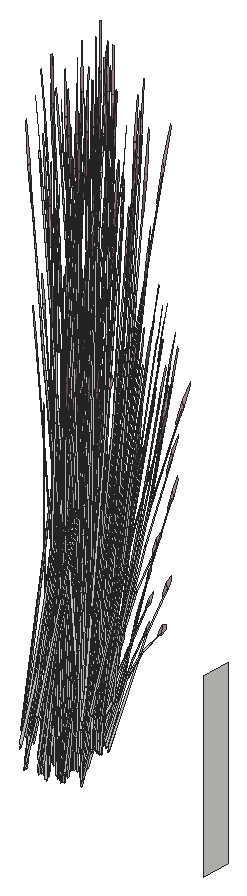
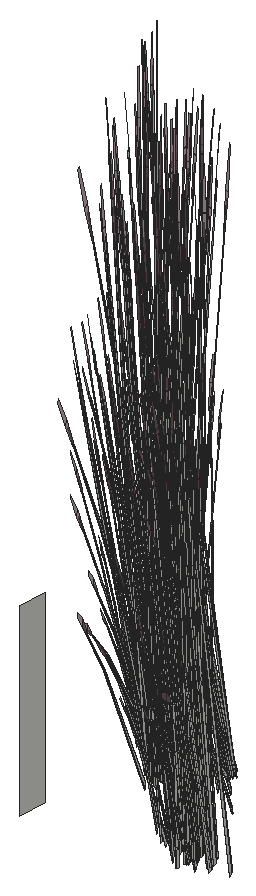
# SketchUp Ruby script. Lengths in inches.
U = 1.inch
M = Sketchup.active_model
def pt(a) = Geom::Point3d.new(a.map { |v| v * U })
def face(e, loops, mat)
  f = e.add_face(loops[0].map { |a| pt(a) })
  loops[1..].each { |l| e.add_face(l.map { |a| pt(a) }).erase! }
  f.material = f.back_material = mat if mat
  f
end
# faces: each face lists its corners as indices into pts; further lists are holes
def faces(e, pts, list, mat = nil) = list.each { |f| face(e, (f[0].is_a?(Array) ? f : [f]).map { |l| l.map { |i| pts[i] } }, mat) }
# xy, xz, yz: faces in a plane at the given z, y or x. An outline is a flat list of corners, or four numbers for a rectangle; further outlines are holes
def ring(l) = l.size == 4 ? [[l[0], l[1]], [l[2], l[1]], [l[2], l[3]], [l[0], l[3]]] : l.each_slice(2).to_a
def flat(e, list, mat, &to3) = list.each { |f| face(e, (f[0].is_a?(Array) ? f : [f]).map { |l| ring(l).map { |u, v| to3.(u, v) } }, mat) }
def xy(e, z, list, mat = nil) = flat(e, list, mat) { |x, y| [x, y, z] }
def xz(e, y, list, mat = nil) = flat(e, list, mat) { |x, z| [x, y, z] }
def yz(e, x, list, mat = nil) = flat(e, list, mat) { |y, z| [x, y, z] }
def lines(e, pts, list) = list.each { |a, b| e.add_line(pt(pts[a]), pt(pts[b])) }
# prism: a flat outline (further loops are holes) pulled along v
def prism(e, loops, v, mat = nil)
  f = face(e, loops, mat); d = Geom::Vector3d.new(v.map { |x| x * U })
  f.pushpull(f.normal.samedirection?(d) ? d.length : -d.length)
end
def box(e, o, s, mat = nil) = prism(e, [[o, [o[0] + s[0], o[1], o[2]], [o[0] + s[0], o[1] + s[1], o[2]], [o[0], o[1] + s[1], o[2]]]], [0, 0, s[2]], mat)
def at(x, y, z, deg = 0) = Geom::Transformation.translation(pt([x, y, z])) * Geom::Transformation.rotation(ORIGIN, Z_AXIS, deg.degrees)
def axes(o, x, y, z) = Geom::Transformation.new([*x, 0, *y, 0, *z, 0, *pt(o).to_a, 1])
def part(name) = M.definitions.add(name)
# library, detail: a bought-in or finely detailed component or shape, given as its bounding box
def library(name, o, s) = part(name).tap { |d| box(d.entities, o, s) }
def detail(e, o, s) = box(e.add_group.entities, o, s)
def put(e, d, t, mat = nil) = e.add_instance(d, t).tap { |i| i.material = mat if mat }
def group(e, t, mat = nil) = e.add_group.tap { |g| g.transformation = t; g.material = mat if mat }.entities
root = M.entities
M.materials.add("LightPink_Translucent").color = [144, 107, 117]
M.materials["LightPink_Translucent"].alpha = 0.75
c1 = part("blade")
p = [[2.15,0.21,22],[0,0.17,0],[0.09,0.45,0],[2.18,0.31,22],[2.29,0.31,22],[0.38,0.45,0],
  [2.48,0.24,33],[2.49,0.24,33],[2.48,0.22,33]]
faces(c1.entities,p,[[0,1,2,3],[4,5,2,3],[6,3,4,7],[8,0,3,6]])
c2 = part("seeds")
p = [[0.3,-0.1,1.38],[-0.01,-0.03,1.59],[-0.01,-0.03,0.03],[0.14,-0.07,-0.07],[0.29,-0.03,3],[0.15,0.01,3.11]]
faces(c2.entities,p,[[0,1,2,3],[1,0,4,5]],"LightPink_Translucent")
c3 = part("blade with seeds")
put(c3.entities,c1,at(0,0,0))
put(c3.entities,c2,axes([2.4,0.25,30.99],[1.5799,-0.05474,1.17369],[-0.12525,1.92788,0.29478],[-0.07173,-0.02425,1.56792]))
p = [[375.57,661.9,618],[375.4,659.16,618],[375.4,659.16,636],[375.57,661.9,636]]
faces(root,p,[[0,1,2,3]])
put(root,c3,axes([358.46,657.71,625.58],[-0.26007,0.1585,0.0643],[-0.12729,-0.28902,0.50621],[0.02512,0.1274,0.77189]))
put(root,c3,axes([360.16,659.93,627.39],[0.04504,0.01251,1.77383],[0.13934,0.41205,-0.16761],[-0.0922,0.10815,0.31391]))
put(root,c3,axes([361.1875,659.42,627.36],[-0.09562,0.42421,-0.51099],[-0.32782,-0.1454,-0.3958],[-0.13199,0.0389,0.97773]))
put(root,c3,axes([357.42,661.35,620.03],[0.08291,0.40636,-0.30978],[-0.32928,0.11539,0.30978],[0.06638,0.04686,1.38974]))
put(root,c3,axes([356.62,662,620.67],[0.35635,-0.30962,-0.29095],[0.23697,0.43749,-0.50002],[0.08792,0.04443,1.59708]))
put(root,c3,axes([359.68,662.6,620.47],[-0.2773,-0.3397,0.17642],[0.27945,-0.32949,0.35086],[-0.03063,0.06937,1.60407]))
put(root,c3,axes([358.72,662.4,620.21],[0,-0.53961,0],[0.44133,0,0],[0,0,1.79456]))
put(root,c3,axes([357.68,661.94,623.05],[-0.30722,0.06665,0.35414],[-0.08112,-0.381,-0.4572],[0.08804,-0.10234,0.87481]))
put(root,c3,axes([360.54,661.24,625.45],[0.14709,-0.21136,1.1486],[0.05804,0.3346,0.84392],[-0.1063,0.05991,0.25299]))
put(root,c3,axes([358.31,662.5,620.43],[0.39767,0.22603,0.24065],[-0.19139,0.46966,0.50002],[0,-0.10827,1.60543]))
put(root,c3,axes([358.51,657.62,622.34],[0.05712,-0.02538,1.76342],[0.34359,0.13968,-0.26939],[0.01005,0.15742,0.30037]))
put(root,c3,axes([358.9375,662.61,620.29],[0,0.53934,-0.05637],[-0.44133,0,0],[0,0.01695,1.79368]))
put(root,c3,axes([358.18,662.18,620.72],[-0.38326,0.02879,0.44739],[-0.03466,-0.47788,-0.21531],[0.06861,-0.04843,1.43643]))
put(root,c3,axes([358.59,657.76,625.37],[-0.1064,0.35863,-0.35414],[-0.31043,-0.1046,0.4572],[0.02846,0.14439,0.87481]))
put(root,c3,axes([358,661.36,620.47],[-0.10196,0.46348,0.17642],[-0.3731,-0.13116,0.35086],[0.06445,-0.00226,1.60407]))
put(root,c3,axes([361.17,659.06,627.71],[0.17758,0.42229,-0.1216],[-0.31518,0.20752,-0.67495],[-0.13282,0.05572,1.02557]))
put(root,c3,axes([361.625,659.95,626.56],[0.08815,-0.14329,1.71376],[0.22258,0.38678,0.13857],[-0.15267,0.17614,0.73262]))
put(root,c3,axes([361.1,660.32,627.21],[-0.30722,0.06665,-0.35414],[-0.08112,-0.381,0.4572],[-0.08804,0.10234,0.87481]))
put(root,c3,axes([355.72,661.72,619.59],[-0.3474,0.18671,1.28929],[-0.11057,-0.53572,0.50096],[0.21332,0.00891,1.46642]))
put(root,c3,axes([360.93,661.45,624.17],[0.04734,0.04659,1.76342],[0.08027,0.4317,-0.26939],[-0.10492,0.09206,0.30037]))
put(root,c3,axes([358.37,658.4,625.56],[0.04474,0.0751,1.74944],[0.36104,0.0295,-0.27667],[0.03631,0.16562,0.14031]))
put(root,c3,axes([359.13,661.39,620.47],[-0.37926,0.12378,0.17642],[-0.09365,-0.46065,0.35086],[0.03382,0.06712,1.60407]))
put(root,c3,axes([357.31,660.89,620.375],[0.22066,-0.46731,0],[0.36918,0.26061,-0.51607],[0.08408,0.05936,1.63711]))
put(root,c3,axes([361.14,660.24,627.41],[-0.08753,-0.42921,0.48003],[0.34336,-0.07449,0.3958],[-0.1012,0.10094,0.9933]))
put(root,c3,axes([357.39,663.67,623.05],[-0.20082,-0.29199,0.35414],[0.2293,-0.2764,-0.4572],[0.1165,0.04206,0.87481]))
put(root,c3,axes([358.55,657.38,625.9],[0.1064,-0.35863,0.35414],[0.31043,0.1046,-0.4572],[0.02846,0.14439,0.87481]))
put(root,c3,axes([358.51,662.06,620.36],[-0.29264,0.42323,0.45755],[-0.34767,-0.3736,0.17955],[0.07055,-0.04224,1.58856]))
put(root,c3,axes([359.01,662.73,620.21],[0.24637,0.30123,0],[-0.24637,0.30123,0],[0,0,1.69266]))
put(root,c3,axes([357.52,661.17,620.02],[0.33032,0.23318,-0.49651],[-0.19744,0.41812,0],[0.07523,0.05311,1.57504]))
put(root,c3,axes([359,662.375,620.72],[0.17124,-0.42022,0.44739],[0.35581,0.20224,-0.21531],[0,0.09687,1.43643]))
put(root,c3,axes([361.07,660.16,627.41],[-0.2423,-0.19613,0.0643],[0.14107,-0.2793,0.50621],[-0.07768,0.0903,0.77189]))
put(root,c3,axes([358.89,662.27,620.38],[-0.44609,-0.09826,0.49198],[0.09078,-0.55493,0.19306],[0.06519,0.05359,1.70813]))
put(root,c3,axes([358.28,663.87,621.93],[-0.06755,-0.39203,-0.03492],[0.31928,-0.09013,-0.15832],[0.06667,0.02485,0.52218]))
put(root,c3,axes([357.72,662.86,623.05],[-0.29332,-0.1301,0.35414],[0.08555,-0.37955,-0.4572],[0.11809,-0.0348,0.87481]))
put(root,c3,axes([361.56,660.3,626.56],[0.06572,-0.16029,1.71376],[0.27569,0.33172,0.13857],[-0.12437,0.20675,0.73262]))
put(root,c3,axes([358.62,657.44,625.83],[0.16845,0.3792,-0.71045],[-0.34676,0.21133,0.08574],[0.03939,0.18322,1.00501]))
put(root,c3,axes([357.03,662.07,620.06],[0.36714,0.07646,-0.62353],[-0.07747,0.47163,-0.16365],[0.10956,0.05715,1.37633]))
put(root,c3,axes([358.6,662.35,620.26],[-0.21881,-0.29821,-0.06488],[0.23965,-0.27324,-0.29416],[0.0679,-0.01924,0.97024]))
put(root,c3,axes([361.3,659.1875,627.73],[0.29332,0.1301,0.35414],[-0.08555,0.37955,-0.4572],[-0.11809,0.0348,0.87481]))
put(root,c3,axes([359.02,662.52,620.21],[0.39487,0,0],[0,0.48281,0],[0,0,1.78407]))
put(root,c3,axes([361.35,660.37,627.36],[0.09067,0.42583,-0.51099],[-0.34336,0.07449,-0.3958],[-0.0984,0.11438,0.97773]))
put(root,c3,axes([358.64,661.99,620.72],[-0.21202,-0.39143,0.44739],[0.32115,-0.27564,-0.21531],[0.06861,0.04843,1.43643]))
put(root,c3,axes([358.25,662.08,620.67],[-0.04113,-0.53214,-0.29095],[0.42835,-0.03218,-0.50002],[0.07543,-0.07088,1.59708]))
put(root,c3,axes([359.15,662.47,620.62],[0.32884,-0.136,0.1448],[0.11516,0.38837,-0.41347],[0,0.08547,1.26744]))
put(root,c3,axes([358.97,658.66,626.49],[0.2439,-0.26754,-0.06488],[0.22348,0.29302,-0.29416],[0.01573,0.08303,0.97024]))
put(root,c3,axes([358.09,660.83,620.77],[-0.11756,0.2374,1.1486],[-0.10105,-0.31895,0.84392],[0.09709,-0.07992,0.25299]))
put(root,c3,axes([360.8125,661.13,627.4],[-0.00877,0.09229,1.74944],[0.24897,0.32105,-0.27667],[-0.06518,0.15182,0.14031]))
put(root,c3,axes([357.95,661.88,622.73],[0.2423,0.19613,0.0643],[-0.14107,0.2793,0.50621],[0.07768,-0.0903,0.77189]))
put(root,c3,axes([357.89,661.8,622.73],[0.08753,0.42921,0.48003],[-0.34336,0.07449,0.3958],[0.1012,-0.10094,0.9933]))
put(root,c3,axes([358.75,657.52,625.53],[0.34695,0.11691,-0.51099],[-0.11892,0.40083,-0.3958],[0.03181,0.16138,0.97773]))
put(root,c3,axes([358.45,657.54,625.88],[0.34538,-0.21713,-0.1216],[0.16972,0.38536,-0.67495],[0.04557,0.16239,1.02557]))
put(root,c3,axes([358.19,660.9,620.03],[0.32928,0.11539,-0.30978],[-0.08291,0.40636,0.30978],[0.06638,-0.04686,1.38974]))
put(root,c3,axes([358.64,661.87,622.71],[-0.0461,-0.00354,1.77383],[-0.19143,-0.37951,-0.16761],[0.07688,-0.12478,0.31391]))
put(root,c3,axes([361.72,660.96,624.7],[-0.33032,-0.23318,-0.49651],[0.19744,-0.41812,0],[-0.07523,-0.05311,1.57504]))
put(root,c3,axes([361.1875,660.0625,627.71],[0.32648,0.25715,-0.1216],[-0.18809,0.3724,-0.67495],[-0.09224,0.12945,1.02557]))
put(root,c3,axes([357.93,661.72,622.53],[0.30722,-0.06665,-0.35414],[0.08112,0.381,0.4572],[0.08804,-0.10234,0.87481]))
put(root,c3,axes([359.9,662.61,620.48],[0,-0.46636,0.49651],[0.39487,0,0],[0,0.10622,1.57504]))
put(root,c3,axes([358.12,660.72,620.02],[0.33032,-0.23318,-0.49651],[0.19744,0.41812,0],[0.07523,-0.05311,1.57504]))
put(root,c3,axes([361.92,661.24,625.05],[-0.22066,0.46731,0],[-0.36918,-0.26061,-0.51607],[-0.08408,-0.05936,1.63711]))
put(root,c3,axes([357.99,662.97,622.73],[0.12963,0.31798,0.0643],[-0.23638,0.15564,0.50621],[0.1042,-0.03071,0.77189]))
put(root,c3,axes([358.78,661.88,620.62],[0.06809,-0.4162,0.1448],[0.33266,0.07225,-0.41347],[0.06054,0.04274,1.26744]))
put(root,c3,axes([357.45,663.86,623.03],[0.0189,-0.47427,-0.1216],[0.35781,0.01296,-0.67495],[0.13781,0.03295,1.02557]))
put(root,c3,axes([357.85,662.98,623.03],[-0.17758,-0.42229,-0.1216],[0.31518,-0.20752,-0.67495],[0.13282,-0.05572,1.02557]))
put(root,c3,axes([357.97,662.86,622.73],[-0.09971,0.42522,0.48003],[-0.32782,-0.1454,0.3958],[0.12892,-0.02555,0.9933]))
put(root,c3,axes([360.65,661.18,628.33],[0.31145,0.12449,-0.06488],[-0.0958,0.38314,-0.29416],[-0.05094,0.05817,0.97024]))
put(root,c3,axes([359.25,661.15,620.48],[-0.33032,-0.23318,0.49651],[0.19744,-0.41812,0],[0.07523,0.05311,1.57504]))
put(root,c3,axes([361.35,660.1,627.73],[0.30722,-0.06665,0.35414],[0.08112,0.381,-0.4572],[-0.08804,0.10234,0.87481]))
put(root,c3,axes([358.96,663.59,620.18],[0.37054,-0.15823,-0.19198],[0.1302,0.45581,0.00008],[0.0409,-0.01749,1.73897]))
put(root,c3,axes([359.42,657.58,625.58],[-0.35104,0.10702,0.48003],[-0.06092,-0.41983,0.3958],[0.08256,0.12373,0.9933]))
put(root,c3,axes([359.35,657.67,625.58],[-0.16041,0.29625,0.0643],[-0.22843,-0.17248,0.50621],[0.07385,0.09498,0.77189]))
put(root,c3,axes([357.83,662.62,622.68],[0.09562,-0.42421,-0.51099],[0.32782,0.1454,-0.3958],[0.13199,-0.0389,0.97773]))
put(root,c3,axes([358.94,656.69,624.72],[-0.08068,-0.14973,1.71376],[0.3728,-0.12606,0.13857],[0.08426,0.23506,0.73262]))
put(root,c3,axes([358.97,662.23,620.21],[0.21202,0.39143,-0.44739],[-0.32115,0.27564,0.21531],[0.06861,0.04843,1.43643]))
put(root,c3,axes([358.66,662.89,620.77],[-0.21807,0.07699,1.1486],[0.10265,-0.31819,0.84392],[0.11568,0.02177,0.25299]))
put(root,c3,axes([362.62,660.13,625.35],[-0.35635,0.30962,-0.29095],[-0.23697,-0.43749,-0.50002],[-0.08792,-0.04443,1.59708]))
put(root,c3,axes([361.64,661.11,627.41],[-0.25132,-0.3182,0.48003],[0.2669,-0.27442,0.3958],[-0.04636,0.14929,0.9933]))
put(root,c3,axes([357.95,661.51,620.59],[-0.12609,-0.01381,1.43002],[-0.12917,-0.37055,-0.30754],[0.1549,-0.10482,0.61141]))
put(root,c3,axes([358.03,662.8125,622.53],[0.29332,0.1301,-0.35414],[-0.08555,0.37955,0.4572],[0.11809,-0.0348,0.87481]))
put(root,c3,axes([361.54,661.08,627.41],[-0.29004,-0.02173,0.0643],[0.00795,-0.32812,0.50621],[-0.03035,0.12569,0.77189]))
put(root,c3,axes([361.64,661.21,627.21],[-0.23881,0.24554,-0.35414],[-0.22606,-0.28036,0.4572],[-0.0344,0.14245,0.87481]))
put(root,c3,axes([358.51,661.67,620.06],[0.23773,-0.35053,-0.62353],[0.29532,0.31785,-0.16365],[0.09526,-0.08744,1.37633]))
put(root,c3,axes([362.86,660.47,624.74],[-0.23773,0.35053,-0.62353],[-0.29532,-0.31785,-0.16365],[-0.09526,0.08744,1.37633]))
put(root,c3,axes([358.18,662.74,619.98],[-0.22732,0.05597,1.41583],[-0.03618,-0.44548,0.08104],[0.15921,-0.06743,0.80566]))
put(root,c3,axes([358.43,662.45,619.49],[-0.01845,-0.0708,1.76342],[0.12793,-0.41416,-0.26939],[0.12905,-0.00596,0.30037]))
put(root,c3,axes([358.55,664.24,622.71],[-0.03191,-0.04083,1.77383],[0.06981,-0.43764,-0.16761],[0.12571,-0.02796,0.31391]))
put(root,c3,axes([359.55,661.36,620.03],[0.08291,0.40636,-0.30978],[-0.32928,0.11539,0.30978],[0.06638,0.04686,1.38974]))
put(root,c3,axes([357.23,662.34,621.875],[-0.14639,0.01056,1.71376],[0.09712,-0.45778,0.13857],[0.20862,0.02831,0.73262]))
put(root,c3,axes([358.75,662.01,620.67],[0.35635,-0.30962,-0.29095],[0.23697,0.43749,-0.50002],[0.08792,0.04443,1.59708]))
put(root,c3,axes([363.02,660.27,625.15],[-0.34464,-0.37536,-0.25192],[0.29,-0.42149,0.5513],[-0.0928,0.04391,1.68216]))
put(root,c3,axes([359.8,661.96,623.05],[-0.30722,0.06665,0.35414],[-0.08112,-0.381,-0.4572],[0.08804,-0.10234,0.87481]))
put(root,c3,axes([357.77,662.77,622.98],[0.31014,-0.20596,-0.71045],[0.17284,0.42397,0.08574],[0.14985,-0.04816,1.00501]))
put(root,c3,axes([359.26,656.99,623.4375],[0.00623,-0.15459,1.43002],[0.29764,-0.17268,-0.30754],[0.09188,0.18503,0.61141]))
put(root,c3,axes([362.85,660.19,624.89],[-0.38326,0.02879,-0.44739],[-0.03466,-0.47788,0.21531],[-0.06861,0.04843,1.43643]))
put(root,c3,axes([358.8125,662.32,622.72],[0.04898,-0.07104,1.74944],[-0.06269,-0.43574,-0.27667],[0.12289,-0.08262,0.14031]))
put(root,c3,axes([357.85,661.74,619.59],[-0.3474,0.18671,1.28929],[-0.11057,-0.53572,0.50096],[0.21332,0.00891,1.46642]))
put(root,c3,axes([362.11,660.99,625.16],[0.33032,0.23318,0.49651],[-0.19744,0.41812,0],[-0.07523,-0.05311,1.57504]))
put(root,c3,axes([358.25,663.4,620.59],[-0.085,-0.1147,1.43002],[0.1106,-0.37943,-0.30754],[0.17198,0.0514,0.61141]))
put(root,c3,axes([360,657.75,623.51],[-0.22633,-0.01463,1.0506],[0.14947,-0.31064,0.58006],[0.08941,0.11036,0.8241]))
put(root,c3,axes([362.59,660.27,625.3],[-0.06809,0.4162,0.1448],[-0.33266,-0.07225,-0.41347],[-0.06054,-0.04274,1.26744]))
put(root,c3,axes([359.44,660.91,620.375],[0.22066,-0.46731,0],[0.36918,0.26061,-0.51607],[0.08408,0.05936,1.63711]))
put(root,c3,axes([363.25,661.43,624.7],[-0.33032,0.23318,-0.49651],[-0.19744,-0.41812,0],[-0.07523,0.05311,1.57504]))
put(root,c3,axes([363.27,661.3,624.875],[-0.21791,-0.46895,-0.05142],[0.36918,-0.26061,0.51607],[-0.09097,0.04465,1.6363]))
put(root,c3,axes([359.52,663.69,623.05],[-0.20082,-0.29199,0.35414],[0.2293,-0.2764,-0.4572],[0.1165,0.04206,0.87481]))
put(root,c3,axes([359.64,661.19,620.02],[0.33032,0.23318,-0.49651],[-0.19744,0.41812,0],[0.07523,0.05311,1.57504]))
put(root,c3,axes([363.17,661.24,624.71],[-0.32928,-0.11539,-0.30978],[0.08291,-0.40636,0.30978],[-0.06638,0.04686,1.38974]))
put(root,c3,axes([361.76,660.86,627.73],[0.23881,-0.24554,0.35414],[0.22606,0.28036,-0.4572],[-0.0344,0.14245,0.87481]))
put(root,c3,axes([363.36,659.5,625.52],[-0.00964,-0.43909,1.41272],[0.43635,0.11382,0.59816],[-0.1032,0.24027,1.3335]))
put(root,c3,axes([360.41,663.89,621.93],[-0.06755,-0.39203,-0.03492],[0.31928,-0.09013,-0.15832],[0.06667,0.02485,0.52218]))
put(root,c3,axes([359.85,662.87,623.05],[-0.29332,-0.1301,0.35414],[0.08555,-0.37955,-0.4572],[0.11809,-0.0348,0.87481]))
put(root,c3,axes([359.16,662.08,620.06],[0.36714,0.07646,-0.62353],[-0.07747,0.47163,-0.16365],[0.10956,0.05715,1.37633]))
put(root,c3,axes([360.73,662.36,620.26],[-0.21881,-0.29821,-0.06488],[0.23965,-0.27324,-0.29416],[0.0679,-0.01924,0.97024]))
put(root,c3,axes([363.12,660.0625,625.35],[0.04113,0.53214,-0.29095],[-0.42835,0.03218,-0.50002],[-0.07543,0.07088,1.59708]))
put(root,c3,axes([359.52,657.32,625.53],[0.34827,-0.11086,-0.51099],[0.06092,0.41983,-0.3958],[0.09354,0.12031,0.97773]))
put(root,c3,axes([360.22,660.84,620.77],[-0.11756,0.2374,1.1486],[-0.10105,-0.31895,0.84392],[0.09709,-0.07992,0.25299]))
put(root,c3,axes([360.08,661.9,622.73],[0.2423,0.19613,0.0643],[-0.14107,0.2793,0.50621],[0.07768,-0.0903,0.77189]))
put(root,c3,axes([360.02,661.82,622.73],[0.08753,0.42921,0.48003],[-0.34336,0.07449,0.3958],[0.1012,-0.10094,0.9933]))
put(root,c3,axes([360.77,661.88,622.71],[-0.0461,-0.00354,1.77383],[-0.19143,-0.37951,-0.16761],[0.07688,-0.12478,0.31391]))
put(root,c3,axes([360.05,661.73,622.53],[0.30722,-0.06665,-0.35414],[0.08112,0.381,0.4572],[0.08804,-0.10234,0.87481]))
put(root,c3,axes([360.12,662.99,622.73],[0.12963,0.31798,0.0643],[-0.23638,0.15564,0.50621],[0.1042,-0.03071,0.77189]))
put(root,c3,axes([359.58,663.875,623.03],[0.0189,-0.47427,-0.1216],[0.35781,0.01296,-0.67495],[0.13781,0.03295,1.02557]))
put(root,c3,axes([359.98,663,623.03],[-0.17758,-0.42229,-0.1216],[0.31518,-0.20752,-0.67495],[0.13282,-0.05572,1.02557]))
put(root,c3,axes([362.24,660.76,625.15],[0.37926,-0.12378,0.17642],[0.09365,0.46065,0.35086],[-0.03382,-0.06712,1.60407]))
put(root,c3,axes([360.09,662.875,622.73],[-0.09971,0.42522,0.48003],[-0.32782,-0.1454,0.3958],[0.12892,-0.02555,0.9933]))
put(root,c3,axes([362.73,660.83,624.875],[-0.35581,-0.20937,0],[0.17124,-0.43505,0],[0,0,1.62707]))
put(root,c3,axes([363.55,661.35,625.05],[0.22066,0.46731,0],[-0.36918,0.26061,-0.51607],[-0.08408,0.05936,1.63711]))
put(root,c3,axes([362.33,661.59,627.41],[-0.26007,0.1585,0.0643],[-0.12729,-0.28902,0.50621],[0.02512,0.1274,0.77189]))
put(root,c3,axes([363.37,660.78,625.15],[0.10196,-0.46348,0.17642],[0.3731,0.13116,0.35086],[-0.06445,0.00226,1.60407]))
put(root,c3,axes([363.19,660.17,625.3],[0.26075,0.2802,0.1448],[-0.2175,0.31612,-0.41347],[-0.06054,0.04274,1.26744]))
put(root,c3,axes([363.1875,659.96,625.4],[0.38326,-0.02879,0.44739],[0.03466,0.47788,-0.21531],[-0.06861,0.04843,1.43643]))
put(root,c3,axes([359.96,662.64,622.68],[0.09562,-0.42421,-0.51099],[0.32782,0.1454,-0.3958],[0.13199,-0.0389,0.97773]))
put(root,c3,axes([363.28,661.0625,625.01],[0.44186,0.15158,0.30756],[-0.11054,0.54181,-0.36492],[-0.07313,0.06781,1.64885]))
put(root,c3,axes([360.78,662.91,620.77],[-0.21807,0.07699,1.1486],[0.10265,-0.31819,0.84392],[0.11568,0.02177,0.25299]))
put(root,c3,axes([363.47,661.03,625.16],[0.33032,-0.23318,0.49651],[0.19744,0.41812,0],[-0.07523,0.05311,1.57504]))
put(root,c3,axes([360.08,661.52,620.59],[-0.12609,-0.01381,1.43002],[-0.12917,-0.37055,-0.30754],[0.1549,-0.10482,0.61141]))
put(root,c3,axes([360.16,662.83,622.53],[0.29332,0.1301,-0.35414],[-0.08555,0.37955,0.4572],[0.11809,-0.0348,0.87481]))
put(root,c3,axes([362.81,660.65,624.88],[-0.11516,-0.40207,0],[0.32884,-0.1408,0],[0,0,1.54371]))
put(root,c3,axes([360.3125,662.76,619.98],[-0.22732,0.05597,1.41583],[-0.03618,-0.44548,0.08104],[0.15921,-0.06743,0.80566]))
put(root,c3,axes([360.56,662.46,619.49],[-0.01845,-0.0708,1.76342],[0.12793,-0.41416,-0.26939],[0.12905,-0.00596,0.30037]))
put(root,c3,axes([360.68,664.25,622.71],[-0.03191,-0.04083,1.77383],[0.06981,-0.43764,-0.16761],[0.12571,-0.02796,0.31391]))
put(root,c3,axes([359.36,662.36,621.875],[-0.14639,0.01056,1.71376],[0.09712,-0.45778,0.13857],[0.20862,0.02831,0.73262]))
put(root,c3,axes([363.27,659.86,624.89],[-0.17124,0.42022,-0.44739],[-0.35581,-0.20224,0.21531],[0,0.09687,1.43643]))
put(root,c3,axes([363.95,659.6,625.15],[-0.2773,-0.3397,0.17642],[0.27945,-0.32949,0.35086],[-0.03063,0.06937,1.60407]))
put(root,c3,axes([359.9,662.79,622.98],[0.31014,-0.20596,-0.71045],[0.17284,0.42397,0.08574],[0.14985,-0.04816,1.00501]))
put(root,c3,axes([363.21,659.62,624.97],[0,0.53934,-0.05637],[-0.44133,0,0],[0,0.01695,1.79368]))
put(root,c3,axes([362.43,661.26,627.73],[0.1064,-0.35863,0.35414],[0.31043,0.1046,-0.4572],[0.02846,0.14439,0.87481]))
put(root,c3,axes([360.94,662.34,622.72],[0.04898,-0.07104,1.74944],[-0.06269,-0.43574,-0.27667],[0.12289,-0.08262,0.14031]))
put(root,c3,axes([363,660.66,624.97],[0.15345,0.53576,-0.06012],[-0.43845,0.18773,0],[0.00536,0.01871,1.72173]))
put(root,c3,axes([364.27,659.96,624.88],[-0.44111,-0.00373,-0.04976],[0,-0.52122,0.49943],[-0.01386,0.11865,1.58352]))
put(root,c3,axes([363.4,658.39,625.15],[-0.37926,0.12378,0.17642],[-0.09365,-0.46065,0.35086],[0.03382,0.06712,1.60407]))
put(root,c3,axes([362.85,662.54,628.33],[0.2439,-0.26754,-0.06488],[0.22348,0.29302,-0.29416],[0.01573,0.08303,0.97024]))
put(root,c3,axes([363.28,659.73,624.9],[0.24637,0.30123,0],[-0.24637,0.30123,0],[0,0,1.69266]))
put(root,c3,axes([363.28,659.38,625.4],[0.17124,-0.42022,0.44739],[0.35581,0.20224,-0.21531],[0,0.09687,1.43643]))
put(root,c3,axes([363.13,660.84,624.88],[0.35581,0.20937,0],[-0.17124,0.43505,0],[0,0,1.74954]))
put(root,c3,axes([363.16,659.28,625.0625],[-0.44609,-0.09826,0.49198],[0.09078,-0.55493,0.19306],[0.06519,0.05359,1.70813]))
put(root,c3,axes([364.18,660.04,624.71],[-0.24637,0.29097,-0.30978],[-0.24637,-0.29097,0.30978],[0,0.09372,1.38974]))
put(root,c3,axes([363.47,659.98,624.78],[0.12941,0.42699,-0.69212],[-0.37279,0.15378,-0.18165],[0.0143,0.14459,1.52773]))
put(root,c3,axes([363.29,659.52,624.89],[0.39487,0,0],[0,0.48281,0],[0,0,1.78407]))
put(root,c3,axes([363.43,659.48,625.3],[0.32884,-0.136,0.1448],[0.11516,0.38837,-0.41347],[0,0.08547,1.26744]))
put(root,c3,axes([363.31,659.51,625.35],[0.39748,0.22252,-0.29095],[-0.19139,0.46966,-0.50002],[0.01249,0.11531,1.59708]))
put(root,c3,axes([364.18,659.61,625.16],[0,-0.46636,0.49651],[0.39487,0,0],[0,0.10622,1.57504]))
put(root,c3,axes([364.35,660.05,624.7],[0,0.46636,-0.49651],[-0.39487,0,0],[0,0.10622,1.57504]))
put(root,c3,axes([363.29,661.46,627.41],[-0.35104,0.10702,0.48003],[-0.06092,-0.41983,0.3958],[0.08256,0.12373,0.9933]))
put(root,c3,axes([363.22,661.54,627.41],[-0.16041,0.29625,0.0643],[-0.22843,-0.17248,0.50621],[0.07385,0.09498,0.77189]))
put(root,c3,axes([363.24,660.59,624.87],[0.37054,-0.15823,-0.19198],[0.1302,0.45581,0.00008],[0.0409,-0.01749,1.73897]))
put(root,c3,axes([363.18,661.2,627.73],[-0.05451,-0.37564,0.35414],[0.31161,-0.09919,-0.4572],[0.0837,0.10765,0.87481]))
put(root,c3,axes([363.25,659.24,624.89],[0.21202,0.39143,-0.44739],[-0.32115,0.27564,0.21531],[0.06861,0.04843,1.43643]))
put(root,c3,axes([363.39,659.04,627.15],[-0.30498,-0.24231,1.38283],[0.32203,-0.37727,0.59665],[0.0984,0.22736,1.33663]))
put(root,c3,axes([362.87,661.73,627.39],[0.00104,-0.05646,1.77383],[0.30246,-0.2491,-0.16761],[0.10506,0.08891,0.31391]))
put(root,c3,axes([363.85,661.01,625.45],[-0.19872,-0.13409,1.1486],[0.2566,-0.13625,0.84392],[0.06921,0.11541,0.25299]))
put(root,c3,axes([363.14,660.87,625.27],[0.00623,-0.15459,1.43002],[0.29764,-0.17268,-0.30754],[0.09188,0.18503,0.61141]))
put(root,c3,axes([363.83,658.37,624.71],[0.08291,0.40636,-0.30978],[-0.32928,0.11539,0.30978],[0.06638,0.04686,1.38974]))
put(root,c3,axes([364.45,659.69,625.06],[0.44133,0,0],[0,0.52122,-0.51607],[0,0.11871,1.63711]))
put(root,c3,axes([363.02,659.02,625.35],[0.35635,-0.30962,-0.29095],[0.23697,0.43749,-0.50002],[0.08792,0.04443,1.59708]))
put(root,c3,axes([363.875,661.625,625.35],[-0.22633,-0.01463,1.0506],[0.14947,-0.31064,0.58006],[0.08941,0.11036,0.8241]))
put(root,c3,axes([363.15,661.4,627.71],[0.21031,-0.39918,-0.1216],[0.30457,0.22997,-0.67495],[0.10587,0.11278,1.02557]))
put(root,c3,axes([363.4,661.2,627.36],[0.34827,-0.11086,-0.51099],[0.06092,0.41983,-0.3958],[0.09354,0.12031,0.97773]))
put(root,c3,axes([363.8,660.69,627.73],[-0.20082,-0.29199,0.35414],[0.2293,-0.2764,-0.4572],[0.1165,0.04206,0.87481]))
put(root,c3,axes([363.92,658.19,624.7],[0.33032,0.23318,-0.49651],[-0.19744,0.41812,0],[0.07523,0.05311,1.57504]))
put(root,c3,axes([363.98,660.96,627.41],[-0.01777,0.35463,0.0643],[-0.26836,-0.00972,0.50621],[0.1028,0.03711,0.77189]))
put(root,c3,axes([363.9,661.51,624.17],[0.02571,-0.06733,1.76342],[0.32373,-0.19829,-0.26939],[0.09815,0.10263,0.30037]))
put(root,c3,axes([364,660.85,627.41],[-0.26024,0.30729,0.48003],[-0.22444,-0.32634,0.3958],[0.1221,0.05668,0.9933]))
put(root,c3,axes([364.68,660.89,626.61],[-0.06755,-0.39203,-0.03492],[0.31928,-0.09013,-0.15832],[0.06667,0.02485,0.52218]))
put(root,c3,axes([363.4375,659.09,624.74],[0.36714,0.07646,-0.62353],[-0.07747,0.47163,-0.16365],[0.10956,0.05715,1.37633]))
put(root,c3,axes([363.36,660.1,626.56],[-0.1311,-0.08035,1.71376],[0.27131,-0.33708,0.13857],[0.16909,0.15206,0.73262]))
put(root,c3,axes([364.39,659.99,627.41],[0.12963,0.31798,0.0643],[-0.23638,0.15564,0.50621],[0.1042,-0.03071,0.77189]))
put(root,c3,axes([364.08,660.85,627.21],[0.20082,0.29199,-0.35414],[-0.2293,0.2764,0.4572],[0.1165,0.04206,0.87481]))
put(root,c3,axes([363.85,660.88,627.71],[0.0189,-0.47427,-0.1216],[0.35781,0.01296,-0.67495],[0.13781,0.03295,1.02557]))
put(root,c3,axes([364.37,659.88,627.41],[-0.09971,0.42522,0.48003],[-0.32782,-0.1454,0.3958],[0.12892,-0.02555,0.9933]))
put(root,c3,axes([364.16,660.6,627.4],[0.07571,-0.00789,1.74944],[0.20767,-0.36231,-0.27667],[0.13467,0.04783,0.14031]))
put(root,c3,axes([365.06,659.91,625.45],[-0.21807,0.07699,1.1486],[0.10265,-0.31819,0.84392],[0.11568,0.02177,0.25299]))
put(root,c3,axes([364.4375,659.83,627.21],[0.29332,0.1301,-0.35414],[-0.08555,0.37955,0.4572],[0.11809,-0.0348,0.87481]))
put(root,c3,axes([363.87,660.65,627.66],[0.35281,0.01123,-0.71045],[-0.0237,0.47284,0.08574],[0.14947,0.0499,1.00501]))
put(root,c3,axes([364.96,661.26,627.39],[-0.03191,-0.04083,1.77383],[0.06981,-0.43764,-0.16761],[0.12571,-0.02796,0.31391]))
put(root,c3,axes([363.64,659.36,626.56],[-0.14639,0.01056,1.71376],[0.09712,-0.45778,0.13857],[0.20862,0.02831,0.73262]))
put(root,c3,axes([364.65,660.42,625.27],[-0.085,-0.1147,1.43002],[0.1106,-0.37943,-0.30754],[0.17198,0.0514,0.61141]))
